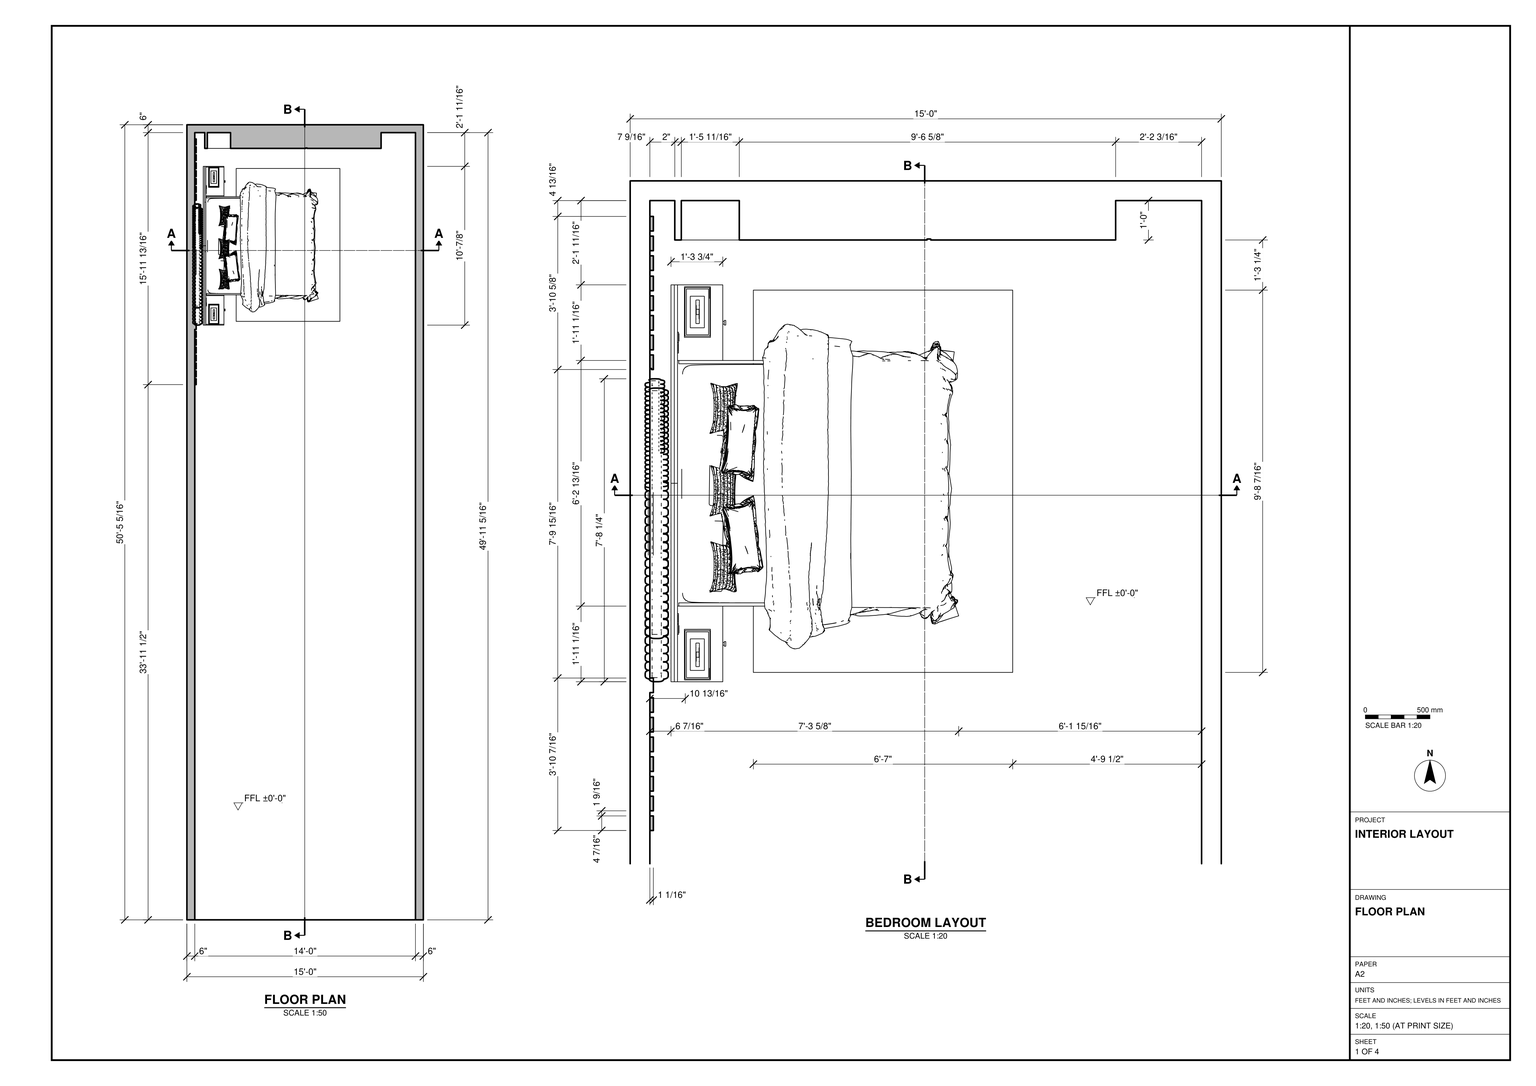
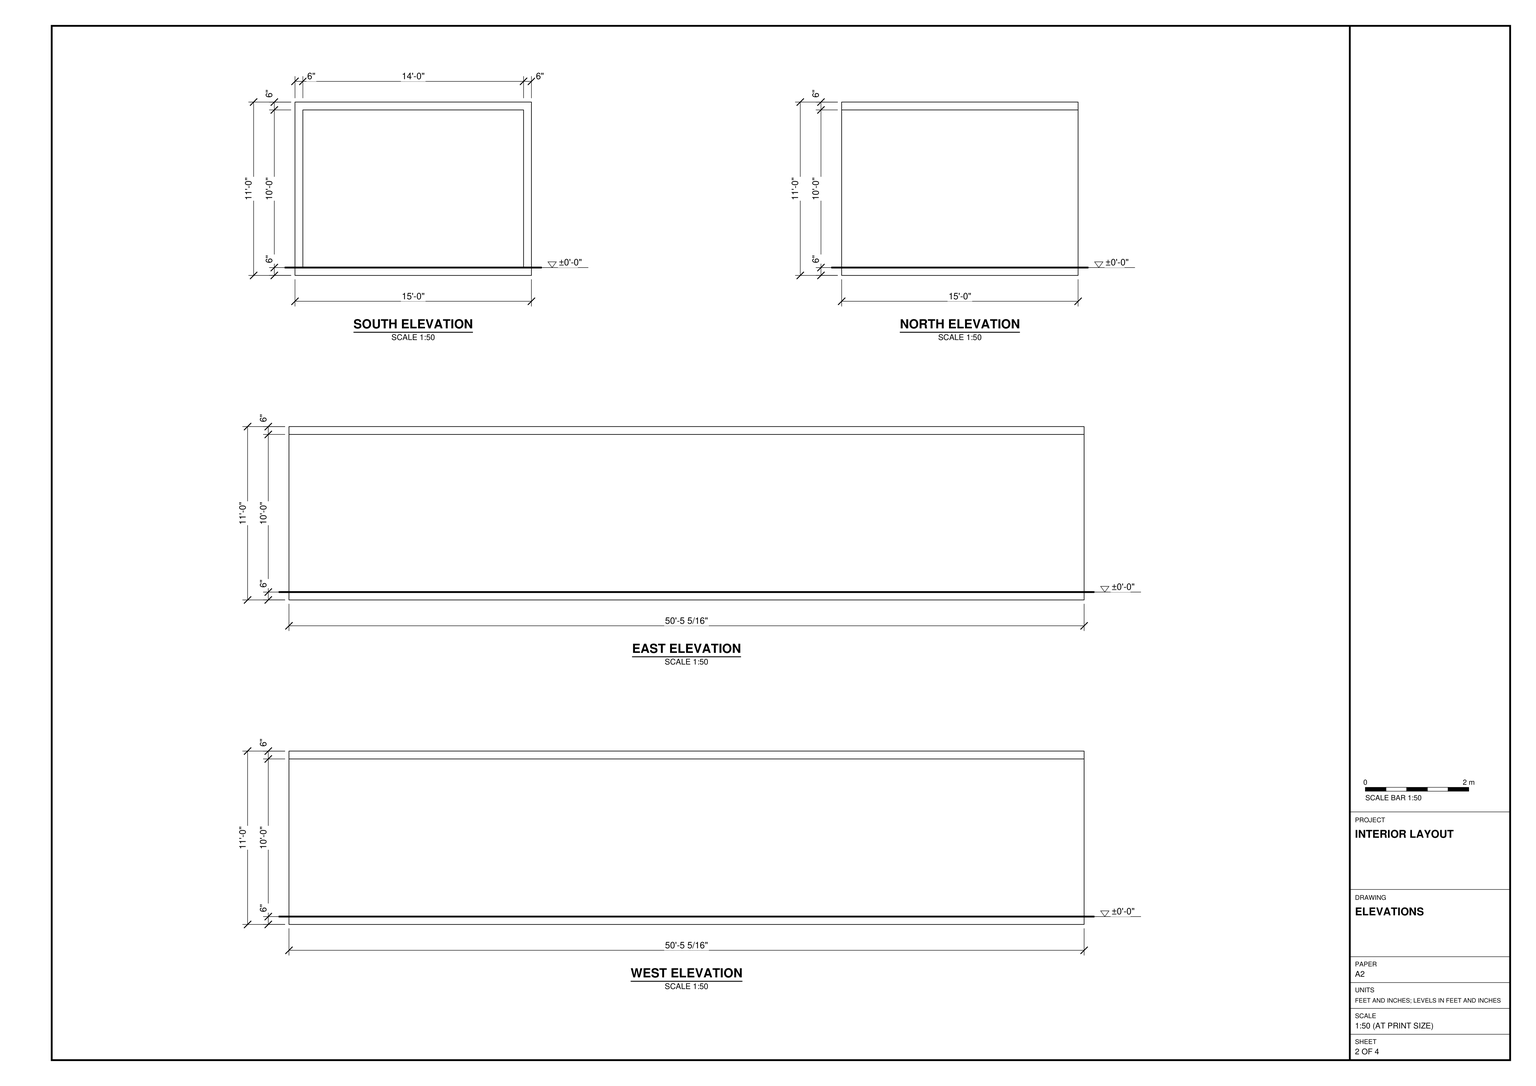
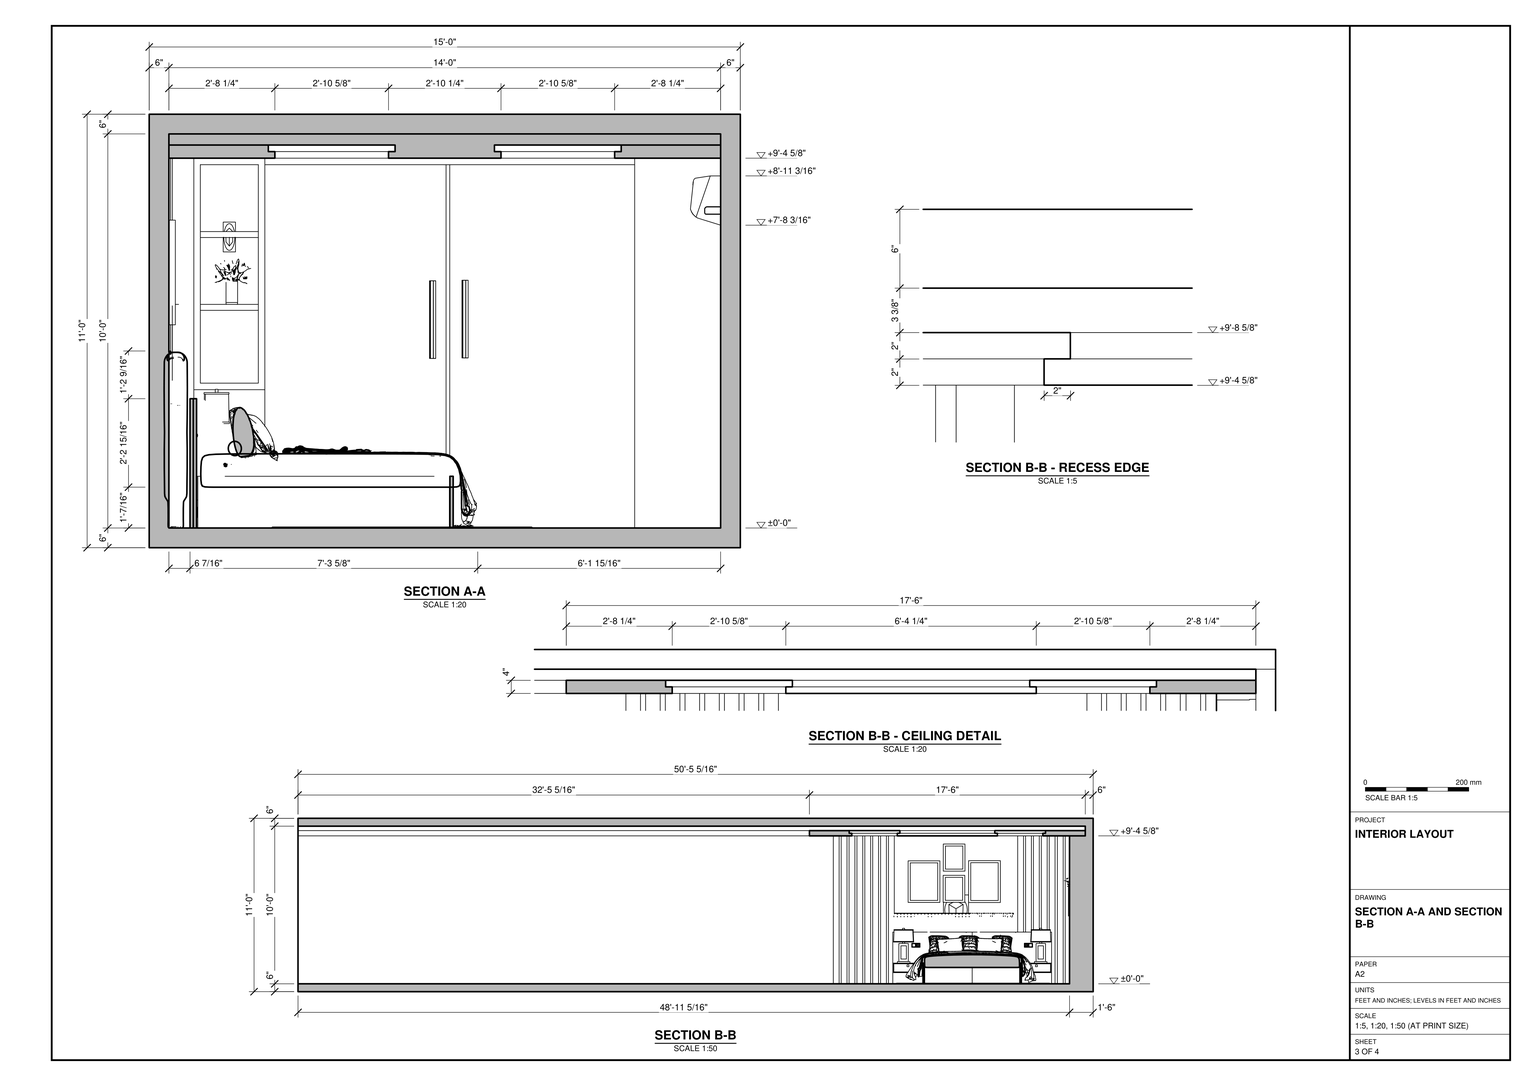
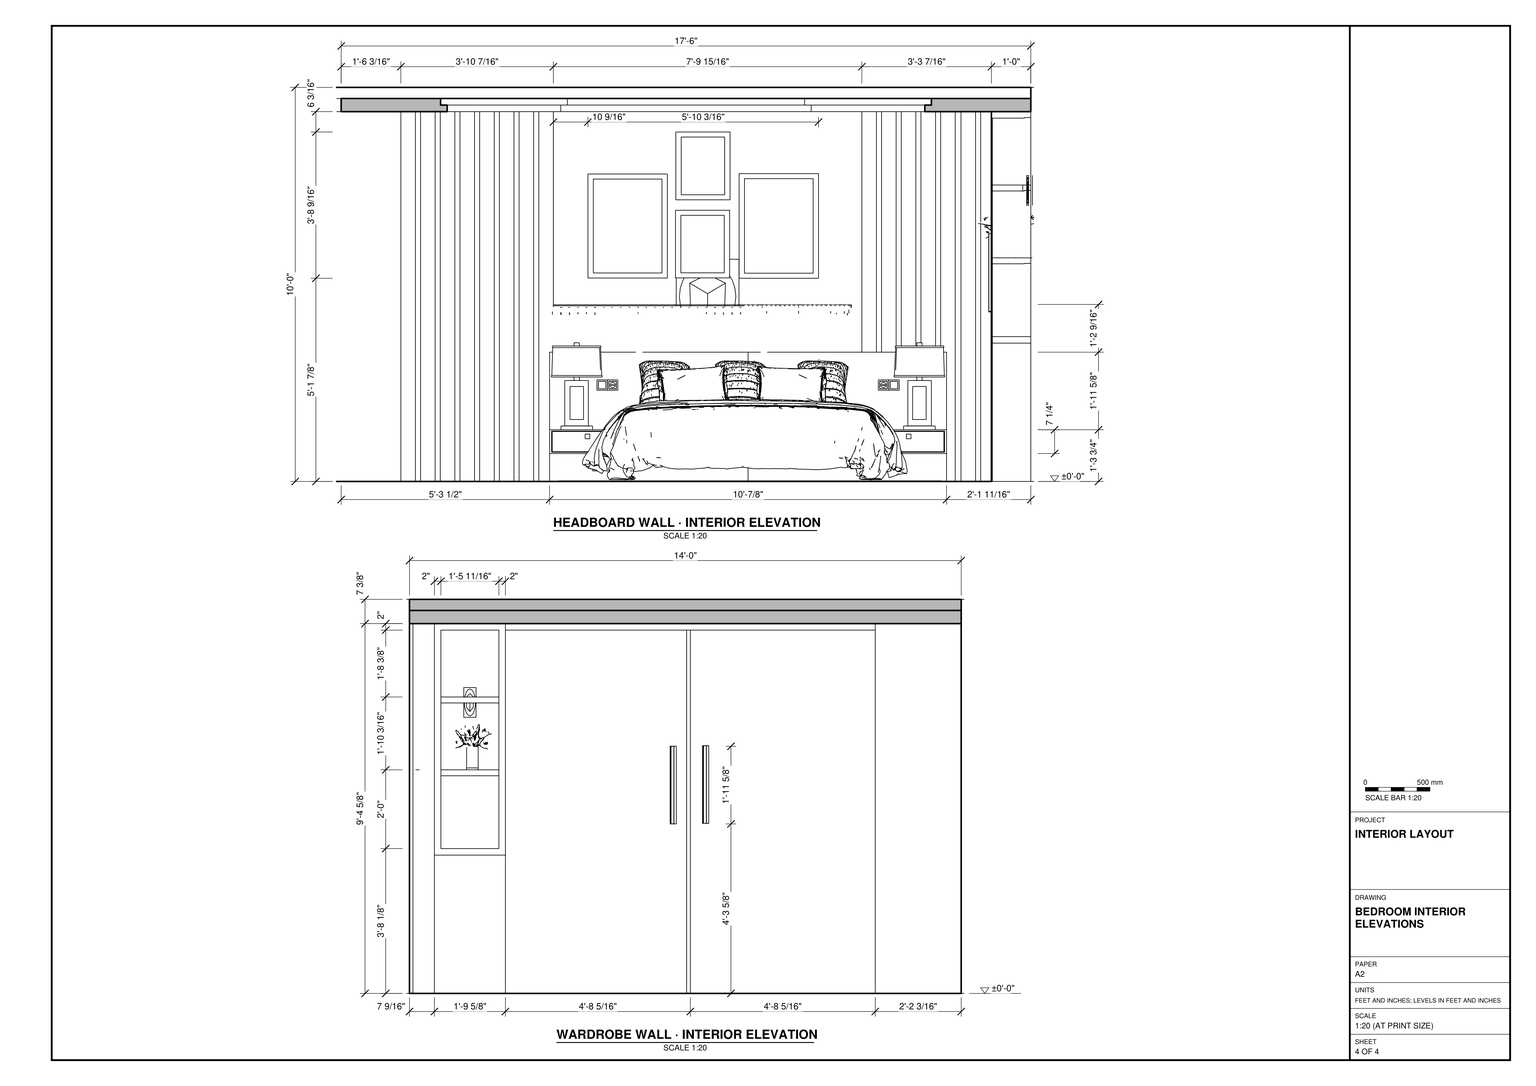
Use task_files/diagram_01.pdf to build the bedroom and its full room shell in SketchUp. Work in feet and inches. The overall model measures 15'-5/8" across, 50'-5 5/16" along its length and 11'-0" high. Set the single finished floor at ±0'-0". Model the 6" side walls, closed north end, floor slab and flat roof slab. Leave the south end open between the side walls as shown in plan and elevation.

Concentrate the fit-out at the north end and leave the long southern portion clear. Place the head of the bed against the west wall with the foot facing east. Use the enlarged bedroom plan to size the bed and bedside tables and to set the clearance beyond the foot. Include the headboard, flanking vertical wall slats, paired wardrobe doors and adjacent open shelving shown in section. Carry the recessed ceiling over the bedroom area only, following the stepped edge profile rather than using a flat panel.

Decor and loose items, including the rug beneath the bed, bedside lamps, bedding and framed pieces above the headboard, may be any suitable library components. Keep the walls, slabs and roof separate, group each furniture or joinery piece separately, and use components for repeated parts. Save one SketchUp model as output_files/bedroom_fit_out_within_its_long_rectangular_shell.skp.

# SketchUp Ruby script. Lengths in inches.
U = 1.inch
M = Sketchup.active_model
def pt(a) = Geom::Point3d.new(a.map { |v| v * U })
def face(e, loops, mat)
  f = e.add_face(loops[0].map { |a| pt(a) })
  loops[1..].each { |l| e.add_face(l.map { |a| pt(a) }).erase! }
  f.material = f.back_material = mat if mat
  f
end
# faces: each face lists its corners as indices into pts; further lists are holes
def faces(e, pts, list, mat = nil) = list.each { |f| face(e, (f[0].is_a?(Array) ? f : [f]).map { |l| l.map { |i| pts[i] } }, mat) }
# xy, xz, yz: faces in a plane at the given z, y or x. An outline is a flat list of corners, or four numbers for a rectangle; further outlines are holes
def ring(l) = l.size == 4 ? [[l[0], l[1]], [l[2], l[1]], [l[2], l[3]], [l[0], l[3]]] : l.each_slice(2).to_a
def flat(e, list, mat, &to3) = list.each { |f| face(e, (f[0].is_a?(Array) ? f : [f]).map { |l| ring(l).map { |u, v| to3.(u, v) } }, mat) }
def xy(e, z, list, mat = nil) = flat(e, list, mat) { |x, y| [x, y, z] }
def xz(e, y, list, mat = nil) = flat(e, list, mat) { |x, z| [x, y, z] }
def yz(e, x, list, mat = nil) = flat(e, list, mat) { |y, z| [x, y, z] }
def lines(e, pts, list) = list.each { |a, b| e.add_line(pt(pts[a]), pt(pts[b])) }
# prism: a flat outline (further loops are holes) pulled along v
def prism(e, loops, v, mat = nil)
  f = face(e, loops, mat); d = Geom::Vector3d.new(v.map { |x| x * U })
  f.pushpull(f.normal.samedirection?(d) ? d.length : -d.length)
end
def box(e, o, s, mat = nil) = prism(e, [[o, [o[0] + s[0], o[1], o[2]], [o[0] + s[0], o[1] + s[1], o[2]], [o[0], o[1] + s[1], o[2]]]], [0, 0, s[2]], mat)
def at(x, y, z, deg = 0) = Geom::Transformation.translation(pt([x, y, z])) * Geom::Transformation.rotation(ORIGIN, Z_AXIS, deg.degrees)
def axes(o, x, y, z) = Geom::Transformation.new([*x, 0, *y, 0, *z, 0, *pt(o).to_a, 1])
def part(name) = M.definitions.add(name)
# library, detail: a bought-in or finely detailed component or shape, given as its bounding box
def library(name, o, s) = part(name).tap { |d| box(d.entities, o, s) }
def detail(e, o, s) = box(e.add_group.entities, o, s)
def put(e, d, t, mat = nil) = e.add_instance(d, t).tap { |i| i.material = mat if mat }
def group(e, t, mat = nil) = e.add_group.tap { |g| g.transformation = t; g.material = mat if mat }.entities
root = M.entities
M.materials.add("Generic").color = [210, 210, 210]
M.materials.add("X22").color = [195, 196, 193]
M.materials.add("[Color M04]").color = [128, 98, 66]
M.materials.add("[Color M05]").color = [202, 158, 102]
M.materials.add("[Color M08]4").color = [30, 30, 30]
M.materials.add("steklo zelenkovatoie1").color = [255, 255, 255]
M.materials["steklo zelenkovatoie1"].alpha = 0.01
M.materials.add("Ìåòàë_ Àëþìèíèé 1").color = [200, 200, 200]
c1 = library("Кровать",[-17.4,-26.33,0],[117.11,127.46,53.91])
c2 = part("X1")
xy(c2.entities,0.79,[[292.49,554.16,383.77,683.125],[106.61,647.12,250.85,858.41],[424.25,648.04,568.45,857.91],[293.37,729.03,384.53,857.56]],"X22")
xy(c2.entities,0.79,[[[281.2,542.875,395.06,694.41],[292.49,554.16,383.77,683.125]],[[95.33,635.84,262.14,869.69],[106.61,647.12,250.85,858.41]],[[412.97,636.75,579.74,869.19],[424.25,648.04,568.45,857.91]],[[282.08,717.74,395.82,868.85],[293.37,729.03,384.53,857.56]]],"[Color M08]4")
xz(c2.entities,542.875,[[281.2,-12.48,395.06,0.79]],"X22")
xz(c2.entities,635.84,[[95.33,-12.48,262.14,0.79]],"X22")
xz(c2.entities,636.75,[[412.97,-12.48,579.74,0.79]],"X22")
xz(c2.entities,694.41,[[281.2,-12.48,395.06,0.79]],"X22")
xz(c2.entities,717.74,[[282.08,-12.48,395.82,0.79]],"X22")
xz(c2.entities,868.85,[[282.08,-12.48,395.82,0.79]],"X22")
xz(c2.entities,869.19,[[412.97,-12.48,579.74,0.79]],"X22")
xz(c2.entities,869.69,[[95.33,-12.48,262.14,0.79]],"X22")
yz(c2.entities,95.33,[[635.84,-12.48,869.69,0.79]],"X22")
yz(c2.entities,262.14,[[635.84,-12.48,869.69,0.79]],"[Color M08]4")
yz(c2.entities,281.2,[[542.875,-12.48,694.41,0.79]],"X22")
yz(c2.entities,282.08,[[717.74,-12.48,868.85,0.79]],"X22")
yz(c2.entities,395.06,[[542.875,-12.48,694.41,0.79]],"X22")
yz(c2.entities,395.82,[[717.74,-12.48,868.85,0.79]],"X22")
yz(c2.entities,412.97,[[636.75,-12.48,869.19,0.79]],"X22")
yz(c2.entities,579.74,[[636.75,-12.48,869.19,0.79]],"X22")
c3 = library("스마트바손잡이",[-0.08,-0.03,8.9],[0.83,23.68,1.89])
c4 = library("Florero",[0,-9.1,0],[22.375,11.9,13.13])
c5 = library("ac+indoor",[0,-9.2,0],[32.28,9.2,11.8125])
c6 = library("Group\#1",[-0.5,-0.5,0],[108.46,150.46,2])
c7 = library("Group\#33",[-0.5,-0.5,0],[1.53,95.54,112.62])
c8 = library("Group\#34",[-0.5,-0.5,0],[18.66,2.94,44.42])
xy(root,-6,[[0,0,180,605.3125]])
xy(root,0,[[6,407.49,7.0625,411.93],[6,413.49,7.0625,417.93],[6,419.49,7.0625,423.93],[6,425.49,7.0625,429.93],[6,431.49,7.0625,435.93],
  [6,437.49,7.0625,441.93],[6,443.49,7.0625,447.93],[6.53,547.86,7.0625,547.86,7.0625,552.3,6,552.3,6,548.16,6.53,548.16],[6,553.86,7.0625,558.3],[6,559.86,7.0625,564.3],
  [6,565.86,7.0625,570.3],[6,571.86,7.0625,576.3],[6,578.05,7.0625,582.49],[6,584.05,7.0625,588.49],[6,590.05,7.0625,594.49]])
xy(root,0,[[6,0,174,0,174,599.3125,147.83,599.3125,147.83,587.3125,91.52,587.3125,91.52,587.61,90.4,587.61,90.4,587.3125,13.59,587.3125,13.59,599.3125,6,599.3125,6,594.49,7.0625,594.49,7.0625,590.05,6,590.05,6,588.49,7.0625,588.49,7.0625,584.05,6,584.05,6,582.49,7.0625,582.49,7.0625,578.05,6,578.05,6,576.3,7.0625,576.3,7.0625,571.86,6,571.86,6,570.3,7.0625,570.3,7.0625,565.86,6,565.86,6,564.3,7.0625,564.3,7.0625,559.86,6,559.86,6,558.3,7.0625,558.3,7.0625,553.86,6,553.86,6,552.3,7.0625,552.3,7.0625,547.86,6.53,547.86,6.53,548.16,6,548.16,6,453.93,7.0625,453.93,7.0625,449.49,6,449.49,6,447.93,7.0625,447.93,7.0625,443.49,6,443.49,6,441.93,7.0625,441.93,7.0625,437.49,6,437.49,6,435.93,7.0625,435.93,7.0625,431.49,6,431.49,6,429.93,7.0625,429.93,7.0625,425.49,6,425.49,6,423.93,7.0625,423.93,7.0625,419.49,6,419.49,6,417.93,7.0625,417.93,7.0625,413.49,6,413.49,6,411.93,7.0625,411.93,7.0625,407.49,6,407.49]],"Generic")
xy(root,44.1,[[15.57,587.3125,33.23,599.3125]],"[Color M04]")
xy(root,52.98,[[6,453.93,6.53,544.68]])
xy(root,53.79,[[6.27,453.625,6.53,544.68]])
xy(root,66.28,[[15.57,587.3125,33.23,597.37]],"[Color M04]")
xy(root,68.09,[[15.57,587.3125,33.23,599.3125]],"[Color M04]")
xy(root,88.46,[[15.57,587.3125,33.23,597.37]],"[Color M04]")
xy(root,90.27,[[15.57,587.3125,33.23,599.3125]],"[Color M04]")
xy(root,110.63,[[90.4,587.3125,91.52,587.61]])
xy(root,110.63,[[15.57,587.3125,33.23,597.37]],"[Color M04]")
xy(root,112.62,[[[6,389.3125,6,407.49,7.0625,407.49,7.0625,411.93,6,411.93,6,413.49,7.0625,413.49,7.0625,417.93,6,417.93,6,419.49,7.0625,419.49,7.0625,423.93,6,423.93,6,425.49,7.0625,425.49,7.0625,429.93,6,429.93,6,431.49,7.0625,431.49,7.0625,435.93,6,435.93,6,437.49,7.0625,437.49,7.0625,441.93,6,441.93,6,443.49,7.0625,443.49,7.0625,447.93,6,447.93,6,449.49,7.0625,449.49,7.0625,453.93,6.53,453.93,6.53,453.625,6,453.625,6,548.16,6.53,548.16,6.53,547.86,7.0625,547.86,7.0625,552.3,6,552.3,6,553.86,7.0625,553.86,7.0625,558.3,6,558.3,6,559.86,7.0625,559.86,7.0625,564.3,6,564.3,6,565.86,7.0625,565.86,7.0625,570.3,6,570.3,6,571.86,7.0625,571.86,7.0625,576.3,6,576.3,6,578.05,7.0625,578.05,7.0625,582.49,6,582.49,6,584.05,7.0625,584.05,7.0625,588.49,6,588.49,6,590.05,7.0625,590.05,7.0625,594.49,6,594.49,6,599.3125,13.59,599.3125,13.59,587.3125,147.83,587.3125,147.83,599.3125,174,599.3125,174,389.3125],[38.27,421.58,141.73,567.04]],[6,407.49,7.0625,411.93],[6,413.49,7.0625,417.93],[6,419.49,7.0625,423.93],[6,425.49,7.0625,429.93],
  [6,431.49,7.0625,435.93],[6,437.49,7.0625,441.93],[6,443.49,7.0625,447.93],[6,449.49,6,453.625,6.53,453.625,6.53,453.93,7.0625,453.93,7.0625,449.49],[72.87,456.18,107.13,532.44],
  [6.53,547.86,6.53,548.16,6,548.16,6,552.3,7.0625,552.3,7.0625,547.86],[6,553.86,7.0625,558.3],[6,559.86,7.0625,564.3],[6,565.86,7.0625,570.3],[6,571.86,7.0625,576.3],
  [6,578.05,7.0625,582.49],[6,584.05,7.0625,588.49],[13.59,587.3125,35.21,599.3125],[35.21,587.3125,147.83,599.3125],[6,590.05,7.0625,594.49]])
xy(root,114.62,[[36.27,419.58,143.73,421.58],[36.27,421.58,38.27,569.04],[141.73,421.58,143.73,567.04],[72.87,456.18,74.87,532.44],[74.87,456.18,107.13,458.18],
  [105.13,458.18,107.13,532.44],[74.87,530.44,105.13,532.44],[38.27,567.04,143.73,569.04]])
xy(root,116.62,[[[6,389.3125,174,599.3125],[36.27,419.58,143.73,569.04]]])
xy(root,116.62,[[[36.27,419.58,143.73,569.04],[74.87,458.18,105.13,530.44]]],"steklo zelenkovatoie1")
xy(root,120,[[6,0,174,599.3125]])
xy(root,126,[[0,0,180,605.3125]])
xz(root,0,[[[0,-6,180,126],[6,0,174,120]],[6,0,174,120]])
xz(root,389.3125,[[6,112.62,174,116.62]])
xz(root,407.49,[[6,0,7.0625,112.62]],"[Color M05]")
xz(root,411.93,[[6,0,7.0625,112.62]],"[Color M05]")
xz(root,413.49,[[6,0,7.0625,112.62]],"[Color M05]")
xz(root,417.93,[[6,0,7.0625,112.62]],"[Color M05]")
xz(root,419.49,[[6,0,7.0625,112.62]],"[Color M05]")
xz(root,421.58,[[38.27,112.62,141.73,114.62]])
xz(root,423.93,[[6,0,7.0625,112.62]],"[Color M05]")
xz(root,425.49,[[6,0,7.0625,112.62]],"[Color M05]")
xz(root,429.93,[[6,0,7.0625,112.62]],"[Color M05]")
xz(root,431.49,[[6,0,7.0625,112.62]],"[Color M05]")
xz(root,435.93,[[6,0,7.0625,112.62]],"[Color M05]")
xz(root,437.49,[[6,0,7.0625,112.62]],"[Color M05]")
xz(root,441.93,[[6,0,7.0625,112.62]],"[Color M05]")
xz(root,443.49,[[6,0,7.0625,112.62]],"[Color M05]")
xz(root,447.93,[[6,0,7.0625,112.62]],"[Color M05]")
xz(root,449.49,[[6,0,7.0625,112.62]],"[Color M05]")
xz(root,453.93,[[6,0,6.53,52.98]])
xz(root,453.93,[[6.53,0,7.0625,112.62]],"[Color M05]")
xz(root,456.18,[[72.87,112.62,107.13,114.62]])
xz(root,532.44,[[72.87,112.62,107.13,114.62]])
xz(root,544.68,[[6,52.98,6,53.49,6.27,53.49,6.27,53.79,6.53,53.79,6.53,52.98]])
xz(root,547.86,[[6.53,0,7.0625,112.62]],"[Color M05]")
xz(root,552.3,[[6,0,7.0625,112.62]],"[Color M05]")
xz(root,553.86,[[6,0,7.0625,112.62]],"[Color M05]")
xz(root,558.3,[[6,0,7.0625,112.62]],"[Color M05]")
xz(root,559.86,[[6,0,7.0625,112.62]],"[Color M05]")
xz(root,564.3,[[6,0,7.0625,112.62]],"[Color M05]")
xz(root,565.86,[[6,0,7.0625,112.62]],"[Color M05]")
xz(root,567.04,[[38.27,112.62,141.73,114.62]])
xz(root,570.3,[[6,0,7.0625,112.62]],"[Color M05]")
xz(root,571.86,[[6,0,7.0625,112.62]],"[Color M05]")
xz(root,576.3,[[6,0,7.0625,112.62]],"[Color M05]")
xz(root,578.05,[[6,0,7.0625,112.62]],"[Color M05]")
xz(root,582.49,[[6,0,7.0625,112.62]],"[Color M05]")
xz(root,584.05,[[6,0,7.0625,112.62]],"[Color M05]")
xz(root,587.3125,[[13.59,0,35.21,42.12],[[13.59,42.12,35.21,112.62],[15.57,44.1,33.23,110.63]],[15.57,66.28,33.23,68.09],[15.57,88.46,33.23,90.27],[35.21,110.63,147.83,112.62]],"[Color M04]")
xz(root,587.3125,[[35.21,0,90.4,110.63],[91.52,0,147.83,110.63]],"Ìåòàë_ Àëþìèíèé 1")
xz(root,587.61,[[90.4,0,91.52,110.63]],"Ìåòàë_ Àëþìèíèé 1")
xz(root,588.49,[[6,0,7.0625,112.62]],"[Color M05]")
xz(root,590.05,[[6,0,7.0625,112.62]],"[Color M05]")
xz(root,594.49,[[6,0,7.0625,112.62]])
xz(root,597.37,[[15.57,66.28,33.23,66.4],[15.57,88.46,33.23,88.64],[15.57,110.63,33.23,110.82]])
xz(root,599.3125,[[6,0,13.59,112.62],[147.83,0,174,112.62],[6,112.62,174,116.62],[6,116.62,174,120]])
xz(root,599.3125,[[15.57,44.1,33.23,66.4],[15.57,68.09,33.23,88.64],[15.57,90.27,33.23,110.82]],"[Color M04]")
xz(root,605.3125,[[0,-6,180,0],[0,0,180,120],[0,120,180,126]])
yz(root,0,[[0,-6,605.3125,0],[0,0,605.3125,120],[0,120,605.3125,126]])
yz(root,6,[[0,0,407.49,112.62],[407.49,0,411.93,112.62],[411.93,0,413.49,112.62],[413.49,0,417.93,112.62],[417.93,0,419.49,112.62],
  [419.49,0,423.93,112.62],[423.93,0,425.49,112.62],[425.49,0,429.93,112.62],[429.93,0,431.49,112.62],[431.49,0,435.93,112.62],
  [435.93,0,437.49,112.62],[437.49,0,441.93,112.62],[441.93,0,443.49,112.62],[443.49,0,447.93,112.62],[447.93,0,449.49,112.62],
  [548.16,0,552.3,112.62],[552.3,0,553.86,112.62],[553.86,0,558.3,112.62],[558.3,0,559.86,112.62],[559.86,0,564.3,112.62],
  [564.3,0,565.86,112.62],[565.86,0,570.3,112.62],[570.3,0,571.86,112.62],[571.86,0,576.3,112.62],[576.3,0,578.05,112.62],
  [578.05,0,582.49,112.62],[582.49,0,584.05,112.62],[584.05,0,588.49,112.62],[588.49,0,590.05,112.62],[590.05,0,594.49,112.62],
  [594.49,0,599.3125,112.62],[0,112.62,389.3125,116.62],[389.3125,112.62,599.3125,116.62],[0,116.62,599.3125,120]])
yz(root,6,[[453.93,0,548.16,0,548.16,112.62,453.625,112.62,453.625,53.49,544.68,53.49,544.68,52.98,453.93,52.98]],"Ìåòàë_ Àëþìèíèé 1")
yz(root,6.27,[[453.625,53.49,544.68,53.79]])
yz(root,6.53,[[547.86,0,548.16,112.62],[453.93,52.98,544.68,53.79],[453.625,53.79,453.93,112.62]])
yz(root,7.0625,[[407.49,0,411.93,112.62],[413.49,0,417.93,112.62],[419.49,0,423.93,112.62],[425.49,0,429.93,112.62],[431.49,0,435.93,112.62],
  [437.49,0,441.93,112.62],[443.49,0,447.93,112.62],[449.49,0,453.93,112.62],[547.86,0,552.3,112.62],[553.86,0,558.3,112.62],
  [559.86,0,564.3,112.62],[565.86,0,570.3,112.62],[571.86,0,576.3,112.62],[578.05,0,582.49,112.62],[584.05,0,588.49,112.62],
  [590.05,0,594.49,112.62]],"[Color M05]")
yz(root,13.59,[[587.3125,0,599.3125,42.12]])
yz(root,13.59,[[587.3125,42.12,599.3125,112.62]],"[Color M04]")
yz(root,15.57,[[587.3125,44.1,599.3125,44.1,599.3125,66.4,597.37,66.4,597.37,66.28,587.3125,66.28],[587.3125,68.09,599.3125,68.09,599.3125,88.64,597.37,88.64,597.37,88.46,587.3125,88.46],[587.3125,90.27,599.3125,90.27,599.3125,110.82,597.37,110.82,597.37,110.63,587.3125,110.63]],"[Color M04]")
yz(root,33.23,[[587.3125,44.1,587.3125,66.28,597.37,66.28,597.37,66.4,599.3125,66.4,599.3125,44.1],[587.3125,68.09,587.3125,88.46,597.37,88.46,597.37,88.64,599.3125,88.64,599.3125,68.09],[587.3125,90.27,587.3125,110.63,597.37,110.63,597.37,110.82,599.3125,110.82,599.3125,90.27]],"[Color M04]")
yz(root,38.27,[[421.58,112.62,567.04,114.62]])
yz(root,72.87,[[456.18,112.62,532.44,114.62]])
yz(root,90.4,[[587.3125,0,587.61,42.12],[587.3125,42.12,587.61,110.63]])
yz(root,91.52,[[587.3125,0,587.61,42.12],[587.3125,42.12,587.61,110.63]])
yz(root,107.13,[[456.18,112.62,532.44,114.62]])
yz(root,141.73,[[421.58,112.62,567.04,114.62]])
yz(root,147.83,[[587.3125,0,599.3125,112.62]],"Ìåòàë_ Àëþìèíèé 1")
yz(root,174,[[0,0,599.3125,112.62],[0,112.62,389.3125,116.62],[389.3125,112.62,599.3125,116.62],[0,116.62,599.3125,120]])
yz(root,180,[[0,-6,605.3125,0],[0,0,605.3125,120],[0,120,605.3125,126]])
put(root,c1,at(16.78,475.82,0))
put(root,c2,axes([7.85,548.48,180.4],[0,-0.14493,0],[0,0,-0.13628],[0.14789,0,0]))
put(root,c3,axes([106.03,587.23,51.8],[0,-1,0],[0,0,1],[-1,0,0]))
put(root,c3,axes([96.15,587.24,51.64],[0,-1,0],[0,0,1],[-1,0,0]))
put(root,c4,axes([7.93,597.99,68.09],[1.04,0,0],[0,1.71,0],[0,0,1.09]))
put(root,c5,axes([174,566.73,92.22],[0,-1.32,0],[1,0,0],[0,0,1.27]))
put(root,c6,at(36.27,419.58,114.62))
put(root,c7,at(6,453.625,0))
put(root,c8,at(15.57,597.37,66.4))
